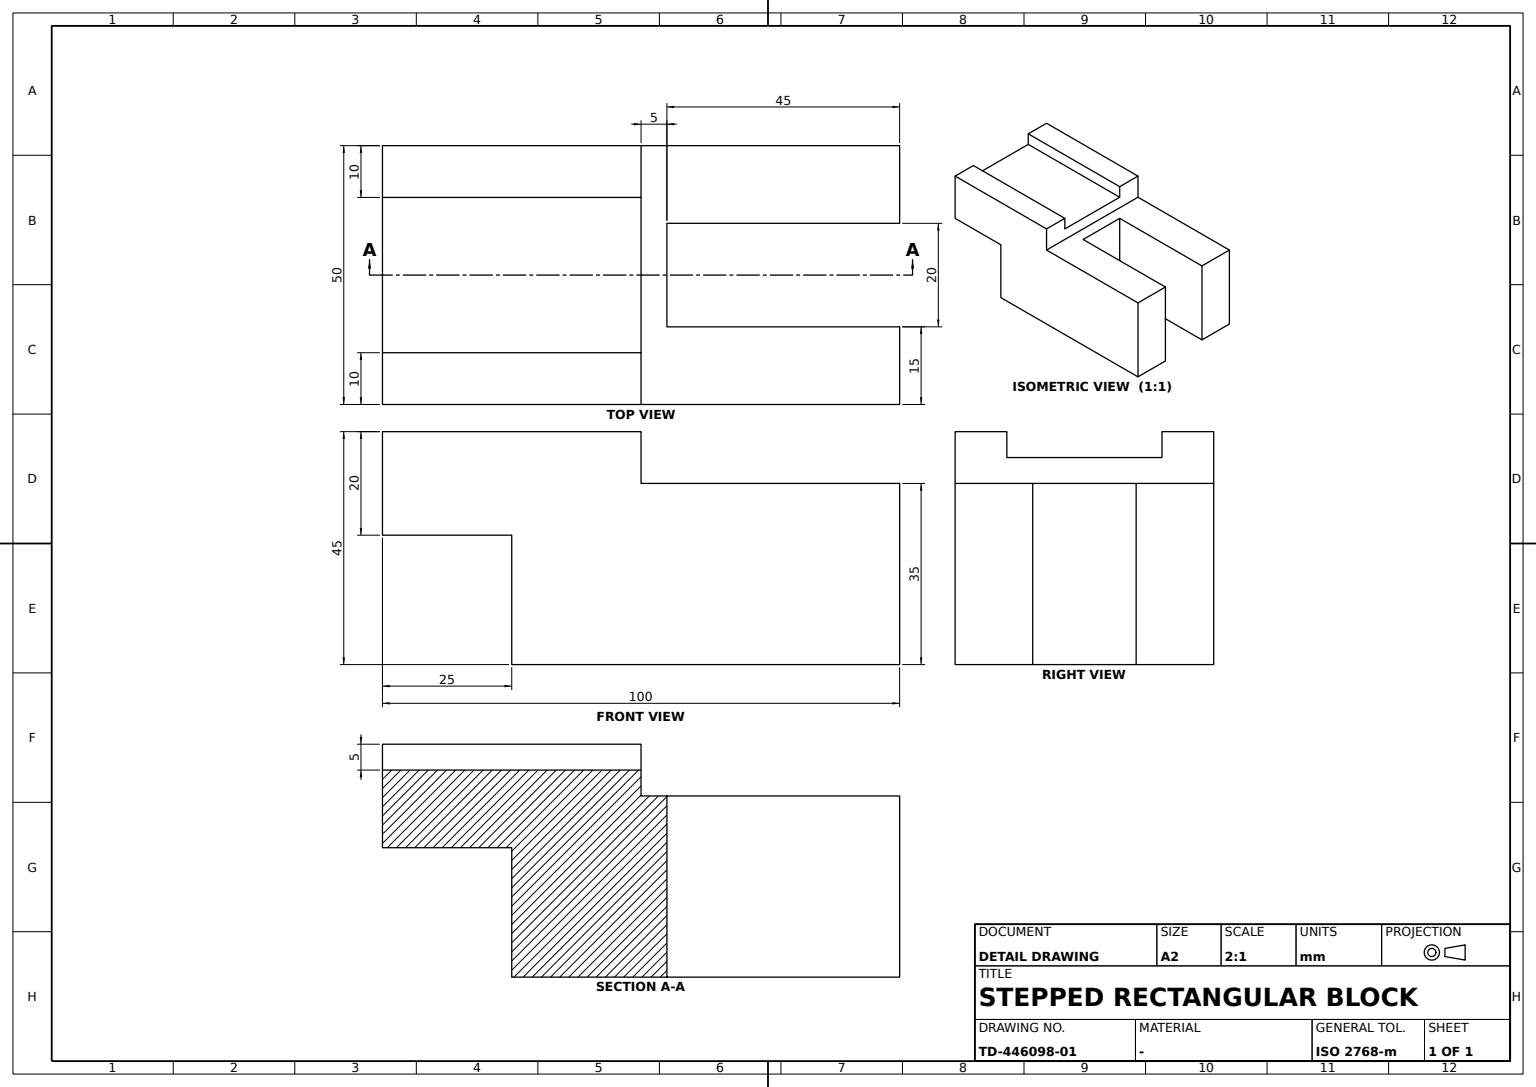
ISO-10303-21;
HEADER;
FILE_DESCRIPTION((''),'2;1');
FILE_NAME('','',(''),(''),'','','');
FILE_SCHEMA(('AUTOMOTIVE_DESIGN'));
ENDSEC;
DATA;
#1=APPLICATION_CONTEXT('');
#2=PRODUCT_CONTEXT('',#1,'mechanical');
#3=PRODUCT('','','',(#2));
#4=PRODUCT_DEFINITION_FORMATION('','',#3);
#5=PRODUCT_DEFINITION_CONTEXT('',#1,'design');
#6=PRODUCT_DEFINITION('','',#4,#5);
#7=PRODUCT_DEFINITION_SHAPE('','',#6);
#8=(LENGTH_UNIT()NAMED_UNIT(*)SI_UNIT(.MILLI.,.METRE.));
#9=(NAMED_UNIT(*)PLANE_ANGLE_UNIT()SI_UNIT($,.RADIAN.));
#10=(NAMED_UNIT(*)SI_UNIT($,.STERADIAN.)SOLID_ANGLE_UNIT());
#11=UNCERTAINTY_MEASURE_WITH_UNIT(LENGTH_MEASURE(0.005),#8,'distance_accuracy_value','');
#12=(GEOMETRIC_REPRESENTATION_CONTEXT(3)GLOBAL_UNCERTAINTY_ASSIGNED_CONTEXT((#11))GLOBAL_UNIT_ASSIGNED_CONTEXT((#8,#9,#10))REPRESENTATION_CONTEXT('',''));
#13=CARTESIAN_POINT('',(0.,0.,17.5));
#14=VERTEX_POINT('',#13);
#15=CARTESIAN_POINT('',(50.,0.,17.5));
#16=VERTEX_POINT('',#15);
#17=CARTESIAN_POINT('',(-50.,0.,17.5));
#18=DIRECTION('',(1.,0.,0.));
#19=VECTOR('',#18,1000.);
#20=LINE('',#17,#19);
#21=EDGE_CURVE('',#14,#16,#20,.T.);
#22=ORIENTED_EDGE('',*,*,#21,.F.);
#23=CARTESIAN_POINT('',(0.,-50.,17.5));
#24=VERTEX_POINT('',#23);
#25=DIRECTION('',(0.,1.,0.));
#26=VECTOR('',#25,1000.);
#27=LINE('',#13,#26);
#28=EDGE_CURVE('',#24,#14,#27,.T.);
#29=ORIENTED_EDGE('',*,*,#28,.F.);
#30=CARTESIAN_POINT('',(50.,-50.,17.5));
#31=VERTEX_POINT('',#30);
#32=CARTESIAN_POINT('',(-50.,-50.,17.5));
#33=LINE('',#32,#19);
#34=EDGE_CURVE('',#24,#31,#33,.T.);
#35=ORIENTED_EDGE('',*,*,#34,.T.);
#36=CARTESIAN_POINT('',(50.,-35.,17.5));
#37=VERTEX_POINT('',#36);
#38=DIRECTION('',(0.,-1.,0.));
#39=VECTOR('',#38,1000.);
#40=LINE('',#15,#39);
#41=EDGE_CURVE('',#37,#31,#40,.T.);
#42=ORIENTED_EDGE('',*,*,#41,.F.);
#43=CARTESIAN_POINT('',(5.,-35.,17.5));
#44=VERTEX_POINT('',#43);
#45=CARTESIAN_POINT('',(-50.,-35.,17.5));
#46=DIRECTION('',(-1.,0.,0.));
#47=VECTOR('',#46,1000.);
#48=LINE('',#45,#47);
#49=EDGE_CURVE('',#37,#44,#48,.T.);
#50=ORIENTED_EDGE('',*,*,#49,.T.);
#51=CARTESIAN_POINT('',(5.,-15.,17.5));
#52=VERTEX_POINT('',#51);
#53=CARTESIAN_POINT('',(5.,0.,17.5));
#54=LINE('',#53,#26);
#55=EDGE_CURVE('',#44,#52,#54,.T.);
#56=ORIENTED_EDGE('',*,*,#55,.T.);
#57=CARTESIAN_POINT('',(50.,-15.,17.5));
#58=VERTEX_POINT('',#57);
#59=LINE('',#57,#47);
#60=EDGE_CURVE('',#58,#52,#59,.T.);
#61=ORIENTED_EDGE('',*,*,#60,.F.);
#62=EDGE_CURVE('',#16,#58,#40,.T.);
#63=ORIENTED_EDGE('',*,*,#62,.F.);
#64=EDGE_LOOP('',(#22,#29,#35,#42,#50,#56,#61,#63));
#65=FACE_BOUND('',#64,.T.);
#66=DIRECTION('',(0.,0.,-1.));
#67=AXIS2_PLACEMENT_3D('',#17,#66,#18);
#68=PLANE('',#67);
#69=ADVANCED_FACE('',(#65),#68,.F.);
#70=CARTESIAN_POINT('',(-50.,-10.,22.5));
#71=VERTEX_POINT('',#70);
#72=CARTESIAN_POINT('',(-50.,-40.,22.5));
#73=VERTEX_POINT('',#72);
#74=LINE('',#70,#39);
#75=EDGE_CURVE('',#71,#73,#74,.T.);
#76=ORIENTED_EDGE('',*,*,#75,.T.);
#77=CARTESIAN_POINT('',(0.,-40.,22.5));
#78=VERTEX_POINT('',#77);
#79=LINE('',#77,#47);
#80=EDGE_CURVE('',#78,#73,#79,.T.);
#81=ORIENTED_EDGE('',*,*,#80,.F.);
#82=CARTESIAN_POINT('',(0.,-10.,22.5));
#83=VERTEX_POINT('',#82);
#84=LINE('',#82,#39);
#85=EDGE_CURVE('',#83,#78,#84,.T.);
#86=ORIENTED_EDGE('',*,*,#85,.F.);
#87=LINE('',#82,#47);
#88=EDGE_CURVE('',#83,#71,#87,.T.);
#89=ORIENTED_EDGE('',*,*,#88,.T.);
#90=EDGE_LOOP('',(#76,#81,#86,#89));
#91=FACE_BOUND('',#90,.T.);
#92=AXIS2_PLACEMENT_3D('',#82,#66,#38);
#93=PLANE('',#92);
#94=ADVANCED_FACE('',(#91),#93,.F.);
#95=ORIENTED_EDGE('',*,*,#60,.T.);
#96=CARTESIAN_POINT('',(5.,-15.,-17.5));
#97=VERTEX_POINT('',#96);
#98=VECTOR('',#66,1000.);
#99=LINE('',#51,#98);
#100=EDGE_CURVE('',#52,#97,#99,.T.);
#101=ORIENTED_EDGE('',*,*,#100,.T.);
#102=CARTESIAN_POINT('',(50.,-15.,-17.5));
#103=VERTEX_POINT('',#102);
#104=LINE('',#102,#47);
#105=EDGE_CURVE('',#103,#97,#104,.T.);
#106=ORIENTED_EDGE('',*,*,#105,.F.);
#107=LINE('',#57,#98);
#108=EDGE_CURVE('',#58,#103,#107,.T.);
#109=ORIENTED_EDGE('',*,*,#108,.F.);
#110=EDGE_LOOP('',(#95,#101,#106,#109));
#111=FACE_BOUND('',#110,.T.);
#112=AXIS2_PLACEMENT_3D('',#57,#25,#66);
#113=PLANE('',#112);
#114=ADVANCED_FACE('',(#111),#113,.F.);
#115=CARTESIAN_POINT('',(-25.,-50.,7.5));
#116=VERTEX_POINT('',#115);
#117=CARTESIAN_POINT('',(-25.,-50.,-17.5));
#118=VERTEX_POINT('',#117);
#119=LINE('',#115,#98);
#120=EDGE_CURVE('',#116,#118,#119,.T.);
#121=ORIENTED_EDGE('',*,*,#120,.F.);
#122=CARTESIAN_POINT('',(-25.,0.,7.5));
#123=VERTEX_POINT('',#122);
#124=LINE('',#122,#39);
#125=EDGE_CURVE('',#123,#116,#124,.T.);
#126=ORIENTED_EDGE('',*,*,#125,.F.);
#127=CARTESIAN_POINT('',(-25.,0.,-17.5));
#128=VERTEX_POINT('',#127);
#129=LINE('',#122,#98);
#130=EDGE_CURVE('',#123,#128,#129,.T.);
#131=ORIENTED_EDGE('',*,*,#130,.T.);
#132=LINE('',#127,#39);
#133=EDGE_CURVE('',#128,#118,#132,.T.);
#134=ORIENTED_EDGE('',*,*,#133,.T.);
#135=EDGE_LOOP('',(#121,#126,#131,#134));
#136=FACE_BOUND('',#135,.T.);
#137=AXIS2_PLACEMENT_3D('',#122,#46,#66);
#138=PLANE('',#137);
#139=ADVANCED_FACE('',(#136),#138,.T.);
#140=ORIENTED_EDGE('',*,*,#41,.T.);
#141=CARTESIAN_POINT('',(50.,-50.,-17.5));
#142=VERTEX_POINT('',#141);
#143=LINE('',#30,#98);
#144=EDGE_CURVE('',#31,#142,#143,.T.);
#145=ORIENTED_EDGE('',*,*,#144,.T.);
#146=CARTESIAN_POINT('',(50.,-35.,-17.5));
#147=VERTEX_POINT('',#146);
#148=CARTESIAN_POINT('',(50.,0.,-17.5));
#149=LINE('',#148,#39);
#150=EDGE_CURVE('',#147,#142,#149,.T.);
#151=ORIENTED_EDGE('',*,*,#150,.F.);
#152=DIRECTION('',(0.,0.,1.));
#153=VECTOR('',#152,1000.);
#154=LINE('',#36,#153);
#155=EDGE_CURVE('',#147,#37,#154,.T.);
#156=ORIENTED_EDGE('',*,*,#155,.T.);
#157=EDGE_LOOP('',(#140,#145,#151,#156));
#158=FACE_BOUND('',#157,.T.);
#159=AXIS2_PLACEMENT_3D('',#15,#46,#66);
#160=PLANE('',#159);
#161=ADVANCED_FACE('',(#158),#160,.F.);
#162=CARTESIAN_POINT('',(0.,-40.,27.5));
#163=VERTEX_POINT('',#162);
#164=LINE('',#77,#153);
#165=EDGE_CURVE('',#78,#163,#164,.T.);
#166=ORIENTED_EDGE('',*,*,#165,.T.);
#167=CARTESIAN_POINT('',(0.,-50.,27.5));
#168=VERTEX_POINT('',#167);
#169=CARTESIAN_POINT('',(0.,0.,27.5));
#170=LINE('',#169,#39);
#171=EDGE_CURVE('',#163,#168,#170,.T.);
#172=ORIENTED_EDGE('',*,*,#171,.T.);
#173=CARTESIAN_POINT('',(0.,-50.,0.));
#174=LINE('',#173,#98);
#175=EDGE_CURVE('',#168,#24,#174,.T.);
#176=ORIENTED_EDGE('',*,*,#175,.T.);
#177=ORIENTED_EDGE('',*,*,#28,.T.);
#178=VERTEX_POINT('',#169);
#179=CARTESIAN_POINT('',(0.,0.,0.));
#180=LINE('',#179,#153);
#181=EDGE_CURVE('',#14,#178,#180,.T.);
#182=ORIENTED_EDGE('',*,*,#181,.T.);
#183=CARTESIAN_POINT('',(0.,-10.,27.5));
#184=VERTEX_POINT('',#183);
#185=EDGE_CURVE('',#178,#184,#170,.T.);
#186=ORIENTED_EDGE('',*,*,#185,.T.);
#187=LINE('',#183,#98);
#188=EDGE_CURVE('',#184,#83,#187,.T.);
#189=ORIENTED_EDGE('',*,*,#188,.T.);
#190=ORIENTED_EDGE('',*,*,#85,.T.);
#191=EDGE_LOOP('',(#166,#172,#176,#177,#182,#186,#189,#190));
#192=FACE_BOUND('',#191,.T.);
#193=AXIS2_PLACEMENT_3D('',#179,#18,#25);
#194=PLANE('',#193);
#195=ADVANCED_FACE('',(#192),#194,.T.);
#196=CARTESIAN_POINT('',(-50.,-40.,27.5));
#197=VERTEX_POINT('',#196);
#198=CARTESIAN_POINT('',(-50.,-50.,27.5));
#199=VERTEX_POINT('',#198);
#200=CARTESIAN_POINT('',(-50.,0.,27.5));
#201=LINE('',#200,#39);
#202=EDGE_CURVE('',#197,#199,#201,.T.);
#203=ORIENTED_EDGE('',*,*,#202,.T.);
#204=LINE('',#167,#47);
#205=EDGE_CURVE('',#168,#199,#204,.T.);
#206=ORIENTED_EDGE('',*,*,#205,.F.);
#207=ORIENTED_EDGE('',*,*,#171,.F.);
#208=LINE('',#162,#47);
#209=EDGE_CURVE('',#163,#197,#208,.T.);
#210=ORIENTED_EDGE('',*,*,#209,.T.);
#211=EDGE_LOOP('',(#203,#206,#207,#210));
#212=FACE_BOUND('',#211,.T.);
#213=AXIS2_PLACEMENT_3D('',#169,#66,#38);
#214=PLANE('',#213);
#215=ADVANCED_FACE('',(#212),#214,.F.);
#216=CARTESIAN_POINT('',(-50.,-10.,27.5));
#217=VERTEX_POINT('',#216);
#218=LINE('',#183,#47);
#219=EDGE_CURVE('',#184,#217,#218,.T.);
#220=ORIENTED_EDGE('',*,*,#219,.F.);
#221=ORIENTED_EDGE('',*,*,#185,.F.);
#222=VERTEX_POINT('',#200);
#223=LINE('',#169,#47);
#224=EDGE_CURVE('',#178,#222,#223,.T.);
#225=ORIENTED_EDGE('',*,*,#224,.T.);
#226=EDGE_CURVE('',#222,#217,#201,.T.);
#227=ORIENTED_EDGE('',*,*,#226,.T.);
#228=EDGE_LOOP('',(#220,#221,#225,#227));
#229=FACE_BOUND('',#228,.T.);
#230=ADVANCED_FACE('',(#229),#214,.F.);
#231=CARTESIAN_POINT('',(5.,-35.,-17.5));
#232=VERTEX_POINT('',#231);
#233=CARTESIAN_POINT('',(5.,0.,-17.5));
#234=LINE('',#233,#39);
#235=EDGE_CURVE('',#97,#232,#234,.T.);
#236=ORIENTED_EDGE('',*,*,#235,.F.);
#237=ORIENTED_EDGE('',*,*,#100,.F.);
#238=ORIENTED_EDGE('',*,*,#55,.F.);
#239=LINE('',#231,#153);
#240=EDGE_CURVE('',#232,#44,#239,.T.);
#241=ORIENTED_EDGE('',*,*,#240,.F.);
#242=EDGE_LOOP('',(#236,#237,#238,#241));
#243=FACE_BOUND('',#242,.T.);
#244=CARTESIAN_POINT('',(5.,0.,0.));
#245=AXIS2_PLACEMENT_3D('',#244,#18,#25);
#246=PLANE('',#245);
#247=ADVANCED_FACE('',(#243),#246,.T.);
#248=VERTEX_POINT('',#148);
#249=LINE('',#15,#98);
#250=EDGE_CURVE('',#16,#248,#249,.T.);
#251=ORIENTED_EDGE('',*,*,#250,.F.);
#252=ORIENTED_EDGE('',*,*,#62,.T.);
#253=ORIENTED_EDGE('',*,*,#108,.T.);
#254=EDGE_CURVE('',#248,#103,#149,.T.);
#255=ORIENTED_EDGE('',*,*,#254,.F.);
#256=EDGE_LOOP('',(#251,#252,#253,#255));
#257=FACE_BOUND('',#256,.T.);
#258=ADVANCED_FACE('',(#257),#160,.F.);
#259=LINE('',#146,#47);
#260=EDGE_CURVE('',#147,#232,#259,.T.);
#261=ORIENTED_EDGE('',*,*,#260,.F.);
#262=ORIENTED_EDGE('',*,*,#150,.T.);
#263=LINE('',#141,#47);
#264=EDGE_CURVE('',#142,#118,#263,.T.);
#265=ORIENTED_EDGE('',*,*,#264,.T.);
#266=ORIENTED_EDGE('',*,*,#133,.F.);
#267=LINE('',#148,#47);
#268=EDGE_CURVE('',#248,#128,#267,.T.);
#269=ORIENTED_EDGE('',*,*,#268,.F.);
#270=ORIENTED_EDGE('',*,*,#254,.T.);
#271=ORIENTED_EDGE('',*,*,#105,.T.);
#272=ORIENTED_EDGE('',*,*,#235,.T.);
#273=EDGE_LOOP('',(#261,#262,#265,#266,#269,#270,#271,#272));
#274=FACE_BOUND('',#273,.T.);
#275=AXIS2_PLACEMENT_3D('',#148,#152,#46);
#276=PLANE('',#275);
#277=ADVANCED_FACE('',(#274),#276,.F.);
#278=CARTESIAN_POINT('',(-50.,0.,7.5));
#279=VERTEX_POINT('',#278);
#280=LINE('',#122,#47);
#281=EDGE_CURVE('',#123,#279,#280,.T.);
#282=ORIENTED_EDGE('',*,*,#281,.F.);
#283=ORIENTED_EDGE('',*,*,#125,.T.);
#284=CARTESIAN_POINT('',(-50.,-50.,7.5));
#285=VERTEX_POINT('',#284);
#286=LINE('',#115,#47);
#287=EDGE_CURVE('',#116,#285,#286,.T.);
#288=ORIENTED_EDGE('',*,*,#287,.T.);
#289=LINE('',#278,#39);
#290=EDGE_CURVE('',#279,#285,#289,.T.);
#291=ORIENTED_EDGE('',*,*,#290,.F.);
#292=EDGE_LOOP('',(#282,#283,#288,#291));
#293=FACE_BOUND('',#292,.T.);
#294=AXIS2_PLACEMENT_3D('',#122,#152,#46);
#295=PLANE('',#294);
#296=ADVANCED_FACE('',(#293),#295,.F.);
#297=LINE('',#216,#98);
#298=EDGE_CURVE('',#217,#71,#297,.T.);
#299=ORIENTED_EDGE('',*,*,#298,.T.);
#300=ORIENTED_EDGE('',*,*,#88,.F.);
#301=ORIENTED_EDGE('',*,*,#188,.F.);
#302=ORIENTED_EDGE('',*,*,#219,.T.);
#303=EDGE_LOOP('',(#299,#300,#301,#302));
#304=FACE_BOUND('',#303,.T.);
#305=AXIS2_PLACEMENT_3D('',#183,#25,#66);
#306=PLANE('',#305);
#307=ADVANCED_FACE('',(#304),#306,.F.);
#308=CARTESIAN_POINT('',(-50.,0.,-17.5));
#309=LINE('',#308,#153);
#310=EDGE_CURVE('',#279,#222,#309,.T.);
#311=ORIENTED_EDGE('',*,*,#310,.F.);
#312=ORIENTED_EDGE('',*,*,#290,.T.);
#313=CARTESIAN_POINT('',(-50.,-50.,-17.5));
#314=LINE('',#313,#153);
#315=EDGE_CURVE('',#285,#199,#314,.T.);
#316=ORIENTED_EDGE('',*,*,#315,.T.);
#317=ORIENTED_EDGE('',*,*,#202,.F.);
#318=LINE('',#72,#153);
#319=EDGE_CURVE('',#73,#197,#318,.T.);
#320=ORIENTED_EDGE('',*,*,#319,.F.);
#321=ORIENTED_EDGE('',*,*,#75,.F.);
#322=ORIENTED_EDGE('',*,*,#298,.F.);
#323=ORIENTED_EDGE('',*,*,#226,.F.);
#324=EDGE_LOOP('',(#311,#312,#316,#317,#320,#321,#322,#323));
#325=FACE_BOUND('',#324,.T.);
#326=AXIS2_PLACEMENT_3D('',#308,#18,#152);
#327=PLANE('',#326);
#328=ADVANCED_FACE('',(#325),#327,.F.);
#329=ORIENTED_EDGE('',*,*,#144,.F.);
#330=ORIENTED_EDGE('',*,*,#34,.F.);
#331=ORIENTED_EDGE('',*,*,#175,.F.);
#332=ORIENTED_EDGE('',*,*,#205,.T.);
#333=ORIENTED_EDGE('',*,*,#315,.F.);
#334=ORIENTED_EDGE('',*,*,#287,.F.);
#335=ORIENTED_EDGE('',*,*,#120,.T.);
#336=ORIENTED_EDGE('',*,*,#264,.F.);
#337=EDGE_LOOP('',(#329,#330,#331,#332,#333,#334,#335,#336));
#338=FACE_BOUND('',#337,.T.);
#339=AXIS2_PLACEMENT_3D('',#173,#25,#46);
#340=PLANE('',#339);
#341=ADVANCED_FACE('',(#338),#340,.F.);
#342=ORIENTED_EDGE('',*,*,#281,.T.);
#343=ORIENTED_EDGE('',*,*,#310,.T.);
#344=ORIENTED_EDGE('',*,*,#224,.F.);
#345=ORIENTED_EDGE('',*,*,#181,.F.);
#346=ORIENTED_EDGE('',*,*,#21,.T.);
#347=ORIENTED_EDGE('',*,*,#250,.T.);
#348=ORIENTED_EDGE('',*,*,#268,.T.);
#349=ORIENTED_EDGE('',*,*,#130,.F.);
#350=EDGE_LOOP('',(#342,#343,#344,#345,#346,#347,#348,#349));
#351=FACE_BOUND('',#350,.T.);
#352=AXIS2_PLACEMENT_3D('',#179,#25,#46);
#353=PLANE('',#352);
#354=ADVANCED_FACE('',(#351),#353,.T.);
#355=ORIENTED_EDGE('',*,*,#240,.T.);
#356=ORIENTED_EDGE('',*,*,#49,.F.);
#357=ORIENTED_EDGE('',*,*,#155,.F.);
#358=ORIENTED_EDGE('',*,*,#260,.T.);
#359=EDGE_LOOP('',(#355,#356,#357,#358));
#360=FACE_BOUND('',#359,.T.);
#361=AXIS2_PLACEMENT_3D('',#146,#38,#152);
#362=PLANE('',#361);
#363=ADVANCED_FACE('',(#360),#362,.F.);
#364=ORIENTED_EDGE('',*,*,#80,.T.);
#365=ORIENTED_EDGE('',*,*,#319,.T.);
#366=ORIENTED_EDGE('',*,*,#209,.F.);
#367=ORIENTED_EDGE('',*,*,#165,.F.);
#368=EDGE_LOOP('',(#364,#365,#366,#367));
#369=FACE_BOUND('',#368,.T.);
#370=AXIS2_PLACEMENT_3D('',#77,#38,#152);
#371=PLANE('',#370);
#372=ADVANCED_FACE('',(#369),#371,.F.);
#373=CLOSED_SHELL('',(#69,#94,#114,#139,#161,#195,#215,#230,#247,#258,#277,#296,#307,#328,#341,#354,#363,#372));
#374=MANIFOLD_SOLID_BREP('',#373);
#375=ADVANCED_BREP_SHAPE_REPRESENTATION('',(#374),#12);
#376=SHAPE_DEFINITION_REPRESENTATION(#7,#375);
ENDSEC;
END-ISO-10303-21;
